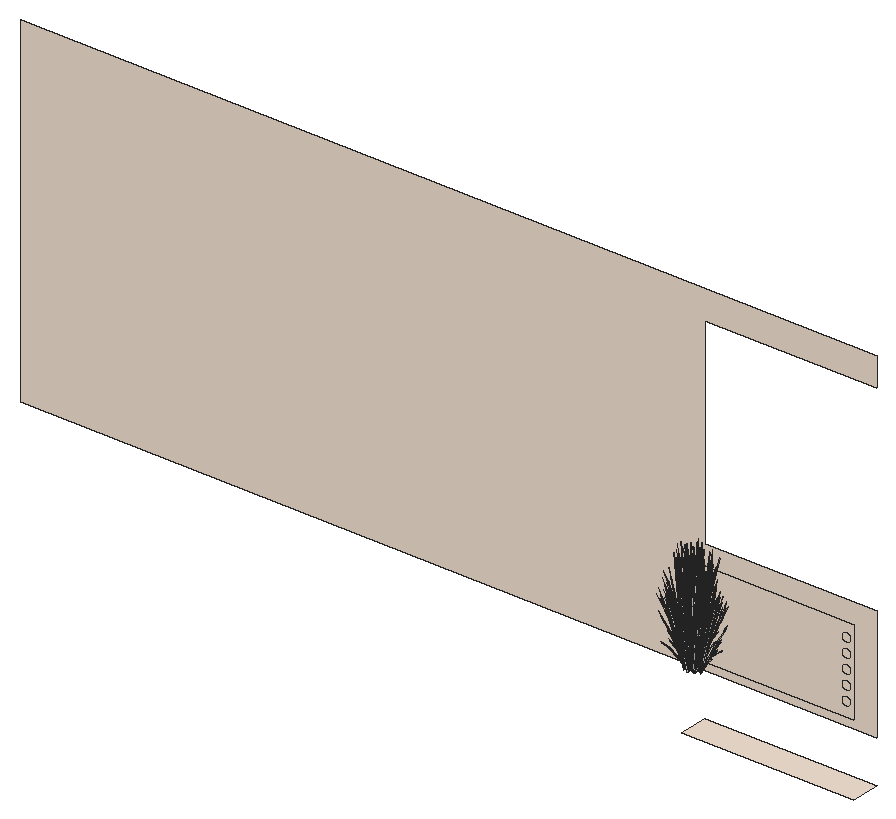
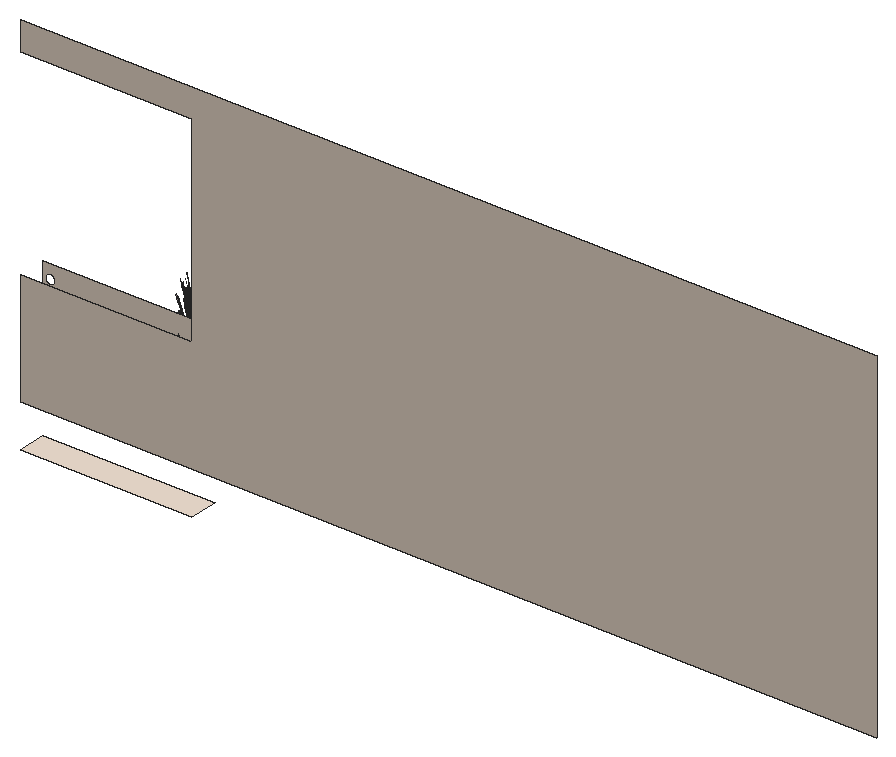
# SketchUp Ruby script. Lengths in inches.
U = 1.inch
M = Sketchup.active_model
def pt(a) = Geom::Point3d.new(a.map { |v| v * U })
def face(e, loops, mat)
  f = e.add_face(loops[0].map { |a| pt(a) })
  loops[1..].each { |l| e.add_face(l.map { |a| pt(a) }).erase! }
  f.material = f.back_material = mat if mat
  f
end
# faces: each face lists its corners as indices into pts; further lists are holes
def faces(e, pts, list, mat = nil) = list.each { |f| face(e, (f[0].is_a?(Array) ? f : [f]).map { |l| l.map { |i| pts[i] } }, mat) }
# xy, xz, yz: faces in a plane at the given z, y or x. An outline is a flat list of corners, or four numbers for a rectangle; further outlines are holes
def ring(l) = l.size == 4 ? [[l[0], l[1]], [l[2], l[1]], [l[2], l[3]], [l[0], l[3]]] : l.each_slice(2).to_a
def flat(e, list, mat, &to3) = list.each { |f| face(e, (f[0].is_a?(Array) ? f : [f]).map { |l| ring(l).map { |u, v| to3.(u, v) } }, mat) }
def xy(e, z, list, mat = nil) = flat(e, list, mat) { |x, y| [x, y, z] }
def xz(e, y, list, mat = nil) = flat(e, list, mat) { |x, z| [x, y, z] }
def yz(e, x, list, mat = nil) = flat(e, list, mat) { |y, z| [x, y, z] }
def lines(e, pts, list) = list.each { |a, b| e.add_line(pt(pts[a]), pt(pts[b])) }
# prism: a flat outline (further loops are holes) pulled along v
def prism(e, loops, v, mat = nil)
  f = face(e, loops, mat); d = Geom::Vector3d.new(v.map { |x| x * U })
  f.pushpull(f.normal.samedirection?(d) ? d.length : -d.length)
end
def box(e, o, s, mat = nil) = prism(e, [[o, [o[0] + s[0], o[1], o[2]], [o[0] + s[0], o[1] + s[1], o[2]], [o[0], o[1] + s[1], o[2]]]], [0, 0, s[2]], mat)
def at(x, y, z, deg = 0) = Geom::Transformation.translation(pt([x, y, z])) * Geom::Transformation.rotation(ORIGIN, Z_AXIS, deg.degrees)
def axes(o, x, y, z) = Geom::Transformation.new([*x, 0, *y, 0, *z, 0, *pt(o).to_a, 1])
def part(name) = M.definitions.add(name)
# library, detail: a bought-in or finely detailed component or shape, given as its bounding box
def library(name, o, s) = part(name).tap { |d| box(d.entities, o, s) }
def detail(e, o, s) = box(e.add_group.entities, o, s)
def put(e, d, t, mat = nil) = e.add_instance(d, t).tap { |i| i.material = mat if mat }
def group(e, t, mat = nil) = e.add_group.tap { |g| g.transformation = t; g.material = mat if mat }.entities
root = M.entities
M.materials.add("C01_Vanilla_Cream").color = [244, 228, 212]
M.materials.add("LightPink_Translucent").color = [144, 107, 117]
M.materials["LightPink_Translucent"].alpha = 0.75
c1 = part("blade")
p = [[2.15,0.21,22],[0,0.17,0],[0.09,0.45,0],[2.18,0.31,22],[2.29,0.31,22],[0.38,0.45,0],
  [2.48,0.24,33],[2.49,0.24,33],[2.48,0.22,33]]
faces(c1.entities,p,[[0,1,2,3],[4,5,2,3],[6,3,4,7],[8,0,3,6]])
c2 = part("seeds")
p = [[0.3,-0.1,1.38],[-0.01,-0.03,1.59],[-0.01,-0.03,0.03],[0.14,-0.07,-0.07],[0.29,-0.03,3],[0.15,0.01,3.11]]
faces(c2.entities,p,[[0,1,2,3],[1,0,4,5]],"LightPink_Translucent")
c3 = part("blade with seeds")
put(c3.entities,c1,at(0,0,0))
put(c3.entities,c2,axes([2.4,0.25,30.99],[1.5799,-0.05474,1.17369],[-0.12525,1.92788,0.29478],[-0.07173,-0.02425,1.56792]))
xy(root,282,[[288,468,360,480]],"C01_Vanilla_Cream")
xz(root,468,[[[288,312,360,348],[357,340,356.48,340.07,356,340.27,355.59,340.59,355.27,341,355.07,341.48,355,342,355.07,342.52,355.27,343,355.59,343.41,356,343.73,356.48,343.93,357,344,357.52,343.93,358,343.73,358.41,343.41,358.73,343,358.93,342.52,359,342,358.93,341.48,358.73,341,358.41,340.59,358,340.27,357.52,340.07],[357,334,356.48,334.07,356,334.27,355.59,334.59,355.27,335,355.07,335.48,355,336,355.07,336.52,355.27,337,355.59,337.41,356,337.73,356.48,337.93,357,338,357.52,337.93,358,337.73,358.41,337.41,358.73,337,358.93,336.52,359,336,358.93,335.48,358.73,335,358.41,334.59,358,334.27,357.52,334.07],[357,328,356.48,328.07,356,328.27,355.59,328.59,355.27,329,355.07,329.48,355,330,355.07,330.52,355.27,331,355.59,331.41,356,331.73,356.48,331.93,357,332,357.52,331.93,358,331.73,358.41,331.41,358.73,331,358.93,330.52,359,330,358.93,329.48,358.73,329,358.41,328.59,358,328.27,357.52,328.07],[357,322,356.48,322.07,356,322.27,355.59,322.59,355.27,323,355.07,323.48,355,324,355.07,324.52,355.27,325,355.59,325.41,356,325.73,356.48,325.93,357,326,357.52,325.93,358,325.73,358.41,325.41,358.73,325,358.93,324.52,359,324,358.93,323.48,358.73,323,358.41,322.59,358,322.27,357.52,322.07],[357,316,356.48,316.07,356,316.27,355.59,316.59,355.27,317,355.07,317.48,355,318,355.07,318.52,355.27,319,355.59,319.41,356,319.73,356.48,319.93,357,320,357.52,319.93,358,319.73,358.41,319.41,358.73,319,358.93,318.52,359,318,358.93,317.48,358.73,317,358.41,316.59,358,316.27,357.52,316.07]]],"C01_Vanilla_Cream")
xz(root,480,[[0,300,0,444,360,444,360,432,288,432,288,348,360,348,360,300]],"C01_Vanilla_Cream")
put(root,c3,axes([301.5625,458.53,315.51],[-0.14302,-0.44985,-0.38324],[0.54163,-0.07869,-0.29685],[0.15522,-0.12083,0.7333]))
put(root,c3,axes([299.2,456.98,313.6],[-0.38473,0.28263,-0.02919],[-0.35252,-0.30954,-0.13237],[-0.02482,-0.08771,0.43661]))
put(root,c3,axes([297.29,457.12,315.54],[-0.11979,-0.00348,1.31208],[-0.38137,0.34775,-0.2075],[-0.20349,-0.07106,0.10523]))
put(root,c3,axes([301.82,458.85,315.78],[-0.515,-0.27165,-0.0912],[0.2967,-0.3934,-0.50621],[0.1455,-0.13675,0.76918]))
put(root,c3,axes([299.69,460.33,314.49],[0.48111,0.19866,1.13446],[-0.47133,0.42798,0.44862],[-0.21112,-0.25366,0.95105]))
put(root,c3,axes([298.68,457.65,315.79],[0.08599,0.39682,0.2656],[-0.49155,0.10478,-0.3429],[-0.13203,-0.11372,0.65611]))
put(root,c3,axes([297.17,458.96,313.51],[0,-0.49266,-0.37238],[0.62289,0,0],[0,-0.11221,1.18128]))
put(root,c3,axes([298.91,457.5,313.51],[0.52105,-0.24633,-0.37238],[0.31144,0.44171,0],[0.11867,-0.0561,1.18128]))
put(root,c3,axes([302,458.35,313.94],[-0.19889,-0.01459,1.07251],[-0.20376,-0.39145,-0.23066],[0.24434,-0.11074,0.45856]))
put(root,c3,axes([297.2,457.91,315.82],[0.45978,-0.36358,0.40322],[0.39653,0.38611,0.33247],[-0.21571,-0.06707,0.83437]))
put(root,c3,axes([303.09,458.73,315.53],[-0.07272,-0.00374,1.33037],[-0.30197,-0.40092,-0.12571],[0.12127,-0.13182,0.23543]))
put(root,c3,axes([299.52,458.51,313.54],[0.375,-0.3703,-0.46765],[0.46584,0.33578,-0.12274],[0.15027,-0.09237,1.03225]))
put(root,c3,axes([302.23,457.63,314.07],[-0.18544,0.25079,0.86145],[-0.15939,-0.33694,0.63294],[0.15316,-0.08443,0.18974]))
put(root,c3,axes([301.96,458.57,315.39],[0.48462,-0.07041,-0.2656],[0.12797,0.4025,0.3429],[0.13888,-0.10811,0.65611]))
put(root,c3,axes([297.41,457.9,315.55],[0.02803,-0.37463,0.04823],[0.42332,0.01027,0.37966],[-0.16216,-0.0392,0.57892]))
put(root,c3,axes([298.87,459.16,313.66],[0.27012,-0.44393,-0.33554],[0.56127,0.21365,0.16149],[0,-0.10233,1.07733]))
put(root,c3,axes([297.25,458.02,315.39],[-0.31678,-0.30846,-0.2656],[0.36171,-0.29199,0.3429],[-0.18378,-0.04443,0.65611]))
put(root,c3,axes([299.12,458.94,314],[-0.06488,-0.56215,-0.21822],[0.6757,-0.03399,-0.37502],[0.11898,-0.07488,1.19781]))
put(root,c3,axes([297.44,458.97,313.52],[0.38863,-0.30738,-0.23233],[0.38863,0.30738,0.23233],[0,-0.09901,1.0423]))
put(root,c3,axes([297.28,457.5,313.6],[-0.1606,0.40228,-0.02919],[-0.4943,-0.12375,-0.13237],[-0.07505,-0.0658,0.43661]))
put(root,c3,axes([301.57,458.8125,315.79],[-0.48462,0.07041,0.2656],[-0.12797,-0.4025,-0.3429],[0.13888,-0.10811,0.65611]))
put(root,c3,axes([298.8,459.53,314],[-0.62699,-0.23507,-0.21822],[0.3019,-0.49615,-0.37502],[-0.0197,-0.12182,1.19781]))
put(root,c3,axes([297.02,459.33,313.78],[-0.69617,0,0],[0,-0.55062,-0.38706],[0,-0.12541,1.22783]))
put(root,c3,axes([297.14,458.35,313.94],[0.1087,0.13716,1.07251],[-0.25048,0.37284,-0.23066],[-0.25719,-0.08912,0.45856]))
put(root,c3,axes([299.03,457.7,313.52],[0.51941,0.1219,-0.23233],[-0.13078,0.42928,0.23233],[0.10471,-0.0495,1.0423]))
put(root,c3,axes([297.59,458.23,315.74],[-0.55654,-0.01186,-0.53284],[0.03738,-0.49951,0.0643],[-0.23578,-0.05271,0.75375]))
put(root,c3,axes([302.01,458.75,315.55],[0.3822,0.20719,0.04823],[-0.22252,0.29505,0.37966],[0.12254,-0.09539,0.57892]))
put(root,c3,axes([301.9,458.66,315.55],[0.13808,0.45342,0.36002],[-0.54163,0.07869,0.29685],[0.15963,-0.10664,0.74497]))
put(root,c3,axes([303.36,459.21,315.54],[0.07726,-0.07504,1.31208],[-0.09888,-0.46032,-0.2075],[0.19384,-0.08728,0.10523]))
put(root,c3,axes([297.56,459.1875,313.75],[-0.51786,0.4142,0.23067],[-0.51817,-0.40984,-0.27369],[-0.01808,-0.11762,1.23664]))
put(root,c3,axes([296.83,457.41,315.53],[0.04127,0.04917,1.33037],[-0.19898,0.44196,-0.12571],[-0.20151,0.0032,0.23543]))
put(root,c3,axes([299.21,459.38,313.82],[0.6273,0.23878,0.18048],[-0.3019,0.49615,0.37502],[0,-0.11437,1.20407]))
put(root,c3,axes([298.96,460.05,313.83],[0.14756,-0.58378,-0.17572],[0.69966,0.10176,0.38453],[-0.12225,-0.08062,1.1733]))
put(root,c3,axes([297.4,458.33,315.51],[-0.40426,0.32635,-0.38324],[-0.35404,-0.34474,-0.29685],[-0.2054,-0.04965,0.7333]))
put(root,c3,axes([297.7,458.18,315.79],[0.31678,0.30846,0.2656],[-0.36171,0.29199,-0.3429],[-0.18378,-0.04443,0.65611]))
put(root,c3,axes([296.49,458.76,314.07],[0.35544,-0.03525,0.86145],[-0.22547,0.31061,0.63294],[-0.17565,-0.04659,0.18974]))
put(root,c3,axes([299,459.05,314.04],[-0.60457,0.03041,0.33554],[-0.05467,-0.50484,-0.16149],[0.10823,-0.05117,1.07733]))
put(root,c3,axes([297.61,457.99,315.78],[-0.02981,0.50103,-0.0912],[-0.56442,-0.01369,-0.50621],[-0.21738,-0.0348,0.76918]))
put(root,c3,axes([297.44,459.42,313.86],[0,0.49266,0.37238],[-0.62289,0,0],[0,-0.11221,1.18128]))
put(root,c3,axes([301.84,459.91,315.78],[-0.28012,-0.44611,-0.0912],[0.49717,-0.21923,-0.50621],[0.20951,-0.05886,0.76918]))
put(root,c3,axes([301.8125,459.53,315.51],[0.15083,-0.44814,-0.38324],[0.51712,0.15361,-0.29685],[0.2082,-0.04109,0.7333]))
put(root,c3,axes([301,457.7,313.78],[0.34808,-0.49367,0],[0.58235,0.27531,-0.38706],[0.13264,0.0627,1.22783]))
put(root,c3,axes([296.9,458.68,314.91],[0.23093,-0.01116,1.28532],[-0.15319,0.4836,0.10393],[-0.32909,-0.02991,0.54946]))
put(root,c3,axes([298.91,459.8125,313.66],[-0.33445,-0.41351,-0.33554],[0.50659,-0.29119,0.16149],[-0.10823,-0.05117,1.07733]))
put(root,c3,axes([298.98,459.23,313.77],[0.24206,0.5509,0.34316],[-0.69162,0.19157,0.13466],[0.00845,-0.10123,1.19142]))
put(root,c3,axes([302.37,459.65,313.49],[-0.35858,0.05912,1.06187],[-0.05708,-0.47061,0.06078],[0.25115,-0.07123,0.60425]))
put(root,c3,axes([303.02,459.24,313.7],[-0.34516,-0.31503,-0.04866],[0.37803,-0.28865,-0.22062],[0.10711,-0.02032,0.72768]))
put(root,c3,axes([298.86,459.66,314.04],[-0.27012,0.44393,0.33554],[-0.56127,-0.21365,-0.16149],[0,-0.10233,1.07733]))
put(root,c3,axes([299.85,459.28,313.65],[0,-0.57005,0],[0.69617,0,0],[0,0,1.34592]))
put(root,c3,axes([300.7,457.96,313.86],[-0.52105,-0.24633,0.37238],[0.31144,-0.44171,0],[0.11867,0.0561,1.18128]))
put(root,c3,axes([301.72,459.6875,315.74],[0.48922,-0.21758,-0.53284],[0.27264,0.44789,0.0643],[0.23638,-0.05088,0.75375]))
put(root,c3,axes([298.61,459.97,313.54],[-0.57914,-0.08077,-0.46765],[0.12221,-0.49823,-0.12274],[-0.17283,-0.06037,1.03225]))
put(root,c3,axes([299.52,458.92,313.77],[-0.46162,0.4471,0.34316],[-0.54842,-0.39467,0.13466],[0.11129,-0.04462,1.19142]))
put(root,c3,axes([300.03,459.72,313.72],[-0.51786,-0.42404,-0.04598],[0.51817,-0.4243,0],[-0.01808,-0.01481,1.31678]))
put(root,c3,axes([298.72,458.18,313.86],[-0.16083,0.48962,0.13232],[-0.58854,-0.13856,0.26315],[0.10167,-0.00238,1.20305]))
put(root,c3,axes([301.64,459.77,315.79],[-0.46269,-0.13744,0.2656],[0.13495,-0.40096,-0.3429],[0.18628,-0.03677,0.65611]))
put(root,c3,axes([296.8,459.04,315.55],[0.15729,-0.44921,0.36002],[0.51712,0.15361,0.29685],[-0.20336,0.027,0.74497]))
put(root,c3,axes([298.48,458.58,313.2],[-0.548,0.19724,0.96696],[-0.17442,-0.56594,0.37572],[0.3365,0.00941,1.09981]))
put(root,c3,axes([299.95,458.73,313.96],[0.1074,-0.43968,0.1086],[0.52474,0.07632,-0.3101],[0.0955,0.04515,0.95058]))
put(root,c3,axes([296.76,458.92,315.55],[-0.20448,-0.33592,0.04823],[0.37288,-0.16442,0.37966],[-0.16437,0.03244,0.57892]))
put(root,c3,axes([299.04,459.77,313.77],[0.70367,0.1038,0.34316],[-0.1432,0.58624,0.13466],[-0.10283,-0.05661,1.19142]))
put(root,c3,axes([302.76,459.34,313.12],[-0.0291,-0.0748,1.32257],[0.20181,-0.43752,-0.20205],[0.20357,-0.00629,0.22528]))
put(root,c3,axes([296.75,459.27,313.12],[0.01412,0.07764,1.32257],[-0.28464,0.40547,-0.20205],[-0.20218,-0.02044,0.22528]))
put(root,c3,axes([299.73,458.84,314.04],[-0.33445,-0.41351,0.33554],[0.50659,-0.29119,-0.16149],[0.10823,0.05117,1.07733]))
put(root,c3,axes([298,460.73,313.52],[-0.13078,-0.42928,-0.23233],[0.51941,-0.1219,0.23233],[-0.10471,-0.0495,1.0423]))
put(root,c3,axes([298.66,460.71,313.86],[0.59825,-0.13076,0.13232],[0.14773,0.48663,0.26315],[-0.05336,-0.0709,1.20305]))
put(root,c3,axes([299.9,458.87,314],[0.56211,-0.32708,-0.21822],[0.3738,0.46216,-0.37502],[0.13869,0.04694,1.19781]))
put(root,c3,axes([302.13,459.73,315.39],[0.46269,0.13744,-0.2656],[-0.13495,0.40096,0.3429],[0.18628,-0.03677,0.65611]))
put(root,c3,axes([297.85,460.92,313.51],[-0.52105,-0.24633,-0.37238],[0.31144,-0.44171,0],[-0.11867,-0.0561,1.18128]))
put(root,c3,axes([301.3125,458,313.51],[0.52105,0.24633,-0.37238],[-0.31144,0.44171,0],[0.11867,0.0561,1.18128]))
put(root,c3,axes([296.69,459.09,315.39],[-0.46269,-0.13744,-0.2656],[0.13495,-0.40096,0.3429],[-0.18628,0.03677,0.65611]))
put(root,c3,axes([300.32,459.4,313.65],[0.62289,0,0],[0,0.51004,0],[0,0,1.33805]))
put(root,c3,axes([299.27,460.05,314],[-0.56211,0.32708,-0.21822],[-0.3738,-0.46216,-0.37502],[-0.13869,-0.04694,1.19781]))
put(root,c3,axes([300.5,458.21,313.86],[-0.59825,0.13076,0.13232],[-0.14773,-0.48663,0.26315],[0.05336,0.0709,1.20305]))
put(root,c3,axes([300.87,459.23,314.91],[-0.23093,0.01116,1.28532],[0.15319,-0.4836,0.10393],[0.32909,0.02991,0.54946]))
put(root,c3,axes([301.17,458.18,313.52],[0.13078,0.42928,-0.23233],[-0.51941,0.1219,0.23233],[0.10471,0.0495,1.0423]))
put(root,c3,axes([302.0625,459.9,315.55],[0.20448,0.33592,0.04823],[-0.37288,0.16442,0.37966],[0.16437,-0.03244,0.57892]))
put(root,c3,axes([300.125,459.14,313.79],[-0.70367,-0.1038,0.36899],[0.1432,-0.58624,0.1448],[0.10283,0.05661,1.2811]))
put(root,c3,axes([302.02,459.78,315.55],[-0.15729,0.44921,0.36002],[-0.51712,-0.15361,0.29685],[0.20336,-0.027,0.74497]))
put(root,c3,axes([299.5625,460.59,313.65],[-0.18165,-0.42474,0],[0.51872,-0.14874,0],[0,0,1.15778]))
put(root,c3,axes([299.22,460.1875,313.96],[-0.1074,0.43968,0.1086],[-0.52474,-0.07632,-0.3101],[-0.0955,-0.04515,0.95058]))
put(root,c3,axes([297.18,459.05,315.79],[0.46269,0.13744,0.2656],[-0.13495,0.40096,-0.3429],[-0.18628,0.03677,0.65611]))
put(root,c3,axes([300.24,460.53,313.64],[0.5845,-0.16716,-0.14398],[0.20539,0.48152,0.00006],[0.06452,-0.01848,1.30423]))
put(root,c3,axes([300.44,460.73,313.86],[0.16083,-0.48962,0.13232],[0.58854,0.13856,0.26315],[-0.10167,0.00238,1.20305]))
put(root,c3,axes([300.3125,459.62,313.66],[0.38863,0.31822,0],[-0.38863,0.31822,0],[0,0,1.2695]))
put(root,c3,axes([298.1,459.02,314.51],[0.15825,-0.07127,1.32798],[0.05457,0.4976,0.10393],[-0.34278,0.06603,0.47463]))
put(root,c3,axes([301.36,459.48,313.86],[-0.43742,-0.35886,0.13232],[0.44081,-0.34807,0.26315],[-0.04831,0.07329,1.20305]))
put(root,c3,axes([300.55,458.94,313.54],[0.57914,0.08077,-0.46765],[-0.12221,0.49823,-0.12274],[0.17283,0.06037,1.03225]))
put(root,c3,axes([303.11,459.8125,314.07],[-0.34399,0.08133,0.86145],[0.16192,-0.33614,0.63294],[0.18249,0.023,0.18974]))
put(root,c3,axes([299.43,460.78,313.65],[-0.56127,-0.22118,0],[0.27012,-0.45959,0],[0,0,1.2203]))
put(root,c3,axes([299.9,460.19,313.85],[-0.54364,-0.39653,-0.18894],[0.45745,-0.44527,0.41347],[-0.14639,0.04639,1.26162]))
put(root,c3,axes([298.47,460.95,313.86],[0.52105,0.24633,0.37238],[-0.31144,0.44171,0],[-0.11867,-0.0561,1.18128]))
put(root,c3,axes([300.31,459.25,314.04],[0.27012,-0.44393,0.33554],[0.56127,0.21365,-0.16149],[0,0.10233,1.07733]))
put(root,c3,axes([302.95,461.23,315.53],[-0.05034,-0.04313,1.33037],[0.11012,-0.46232,-0.12571],[0.1983,-0.02954,0.23543]))
put(root,c3,axes([296.4,459.36,315.54],[-0.09091,0.06396,1.31208],[0.00773,0.46734,-0.2075],[-0.20839,0.06078,0.10523]))
put(root,c3,axes([300.2,459.5,313.72],[0,0.56976,-0.04228],[-0.69617,0,0],[0,0.01791,1.34526]))
put(root,c3,axes([297.01,459.3,315.51],[-0.15083,0.44814,-0.38324],[-0.51712,-0.15361,-0.29685],[-0.2082,0.04109,0.7333]))
put(root,c3,axes([296.99,458.91,315.78],[0.28012,0.44611,-0.0912],[-0.49717,0.21923,-0.50621],[-0.20951,0.05886,0.76918]))
put(root,c3,axes([300.25,459.1,313.66],[0.33445,0.41351,-0.33554],[-0.50659,0.29119,0.16149],[0.10823,0.05117,1.07733]))
put(root,c3,axes([302.51,460.85,314.95],[-0.10656,-0.41414,-0.02619],[0.50364,-0.09521,-0.11874],[0.10517,0.02626,0.39164]))
put(root,c3,axes([298.17,461.21,313.78],[-0.34808,0.49367,0],[-0.58235,-0.27531,-0.38706],[-0.13264,-0.0627,1.22783]))
put(root,c3,axes([301.21,460.84,315.78],[0.02981,-0.50103,-0.0912],[0.56442,0.01369,-0.50621],[0.21738,0.0348,0.76918]))
put(root,c3,axes([301.72,459.5,313.86],[0,-0.49266,0.37238],[0.62289,0,0],[0,0.11221,1.18128]))
put(root,c3,axes([300.16,459.87,314.04],[0.60457,-0.03041,0.33554],[0.05467,0.50484,-0.16149],[-0.10823,0.05117,1.07733]))
put(root,c3,axes([300.54,459.35,313.96],[0.51872,-0.14368,0.1086],[0.18165,0.41027,-0.3101],[0,0.09029,0.95058]))
put(root,c3,axes([301.12,460.64,315.79],[-0.31678,-0.30846,0.2656],[0.36171,-0.29199,-0.3429],[0.18378,0.04443,0.65611]))
put(root,c3,axes([299.625,460.11,313.66],[-0.60457,0.03041,-0.33554],[-0.05467,-0.50484,0.16149],[-0.10823,0.05117,1.07733]))
put(root,c3,axes([302.47,460.35,313.94],[-0.13408,-0.12117,1.07251],[0.17446,-0.40083,-0.23066],[0.27128,0.0543,0.45856]))
put(root,c3,axes([300.07,460.79,313.65],[0.56127,0.22118,0],[-0.27012,0.45959,0],[0,0,1.31215]))
put(root,c3,axes([301.7,460.54,315.54],[0.11943,-0.00833,1.31208],[0.32759,-0.38275,-0.2075],[0.21244,0.05052,0.10523]))
put(root,c3,axes([300.29,461.28,313.64],[-0.34375,-0.4954,-0.03857],[0.58235,-0.27531,0.38706],[-0.1435,0.04717,1.22723]))
put(root,c3,axes([300.17,460.08,313.96],[0.41131,0.296,0.1086],[-0.34309,0.33395,-0.3101],[-0.0955,0.04515,0.95058]))
put(root,c3,axes([296.92,460.16,315.55],[-0.13808,-0.45342,0.36002],[0.54163,-0.07869,0.29685],[-0.15963,0.10664,0.74497]))
put(root,c3,axes([296.82,460.07,315.55],[-0.3822,-0.20719,0.04823],[0.22252,-0.29505,0.37966],[-0.12254,0.09539,0.57892]))
put(root,c3,axes([296.99,459.53,314.91],[0.19317,-0.10421,1.28532],[0.16263,0.48153,0.10393],[-0.30326,0.10883,0.54946]))
put(root,c3,axes([301.24,460.6,315.74],[0.55654,0.01186,-0.53284],[-0.03738,0.49951,0.0643],[0.23578,0.05271,0.75375]))
put(root,c3,axes([300.61,461,313.86],[0.52105,-0.24633,0.37238],[0.31144,0.44171,0],[-0.11867,0.0561,1.18128]))
put(root,c3,axes([299.87,460.61,313.72],[0.24206,0.56598,-0.04509],[-0.69162,0.19832,0],[0.00845,0.01976,1.2913]))
put(root,c3,axes([300.14,461.22,313.52],[-0.51941,-0.1219,-0.23233],[0.13078,-0.42928,0.23233],[-0.10471,0.0495,1.0423]))
put(root,c3,axes([296.39,460.35,313.94],[0.19348,0.04044,1.07251],[0.1247,0.41309,-0.23066],[-0.26282,0.07733,0.45856]))
put(root,c3,axes([297.26,460.01,315.79],[0.48462,-0.07041,0.2656],[0.12797,0.4025,-0.3429],[-0.13888,0.10811,0.65611]))
put(root,c3,axes([302.15,459.58,313.78],[0.69617,0,0],[0,0.55062,-0.38706],[0,0.12541,1.22783]))
put(root,c3,axes([295.39,459.83,315.53],[0.07105,0.01321,1.33037],[0.2198,0.43529,-0.12571],[-0.14545,0.11425,0.23543]))
put(root,c3,axes([301.87,459.86,313.65],[-0.69582,-0.00394,-0.03732],[0,-0.55062,0.37457],[-0.02187,0.12535,1.18764]))
put(root,c3,axes([300.36,459.38,314],[0.62699,0.23507,-0.21822],[-0.3019,0.49615,-0.37502],[0.0197,0.12182,1.19781]))
put(root,c3,axes([295.99,461.21,314.07],[0.23202,-0.22328,0.86145],[0.09155,0.35348,0.63294],[-0.16768,0.06329,0.18974]))
put(root,c3,axes([301.57,460.8,315.39],[0.31678,0.30846,-0.2656],[-0.36171,0.29199,0.3429],[0.18378,0.04443,0.65611]))
put(root,c3,axes([301.72,459.94,313.52],[-0.38863,0.30738,-0.23233],[-0.38863,-0.30738,0.23233],[0,0.09901,1.0423]))
put(root,c3,axes([300.05,459.97,314],[0.06488,0.56215,-0.21822],[-0.6757,0.03399,-0.37502],[-0.11898,0.07488,1.19781]))
put(root,c3,axes([301.41,460.92,315.55],[-0.02803,0.37463,0.04823],[-0.42332,-0.01027,0.37966],[0.16216,0.0392,0.57892]))
put(root,c3,axes([300.3,459.75,313.66],[-0.27012,0.44393,-0.33554],[-0.56127,-0.21365,0.16149],[0,0.10233,1.07733]))
put(root,c3,axes([296.86,460.25,315.39],[-0.48462,0.07041,-0.2656],[-0.12797,-0.4025,0.3429],[-0.13888,0.10811,0.65611]))
put(root,c3,axes([301.45,460.8,315.55],[-0.41051,0.32462,0.36002],[-0.35404,-0.34474,0.29685],[0.1926,0.05988,0.74497]))
put(root,c3,axes([296.16,461.15,316.23],[0.49129,0.13151,-0.04866],[-0.15113,0.40475,-0.22062],[-0.08035,0.06145,0.72768]))
put(root,c3,axes([299.64,460.4,313.54],[-0.375,0.3703,-0.46765],[-0.46584,-0.33578,-0.12274],[-0.15027,0.09237,1.03225]))
put(root,c3,axes([300.14,461.18,315.79],[-0.08599,-0.39682,0.2656],[0.49155,-0.10478,-0.3429],[0.13203,0.11372,0.65611]))
put(root,c3,axes([300.31,461.03,313.75],[0.697,0.16013,0.23067],[-0.17437,0.57237,-0.27369],[-0.11536,0.07164,1.23664]))
put(root,c3,axes([300.26,461.41,313.51],[-0.52105,0.24633,-0.37238],[-0.31144,-0.44171,0],[-0.11867,0.0561,1.18128]))
put(root,c3,axes([301.99,459.96,313.51],[0,0.49266,-0.37238],[-0.62289,0,0],[0,0.11221,1.18128]))
put(root,c3,axes([300.43,460.01,314.91],[-0.2068,-0.08488,1.28532],[0.42797,-0.35609,0.10393],[0.26673,0.16064,0.54946]))
put(root,c3,axes([300.47,458.89,315.36],[-0.48108,-0.25598,1.03712],[0.50798,-0.39855,0.44749],[0.15521,0.24018,1.00248]))
put(root,c3,axes([297.01,459.97,315.78],[0.515,0.27165,-0.0912],[-0.2967,0.3934,-0.50621],[-0.1455,0.13675,0.76918]))
put(root,c3,axes([301.2,460.98,314.07],[-0.31347,-0.14166,0.86145],[0.40476,-0.14393,0.63294],[0.10917,0.12192,0.18974]))
put(root,c3,axes([300.1,461.38,315.78],[0.33176,-0.4217,-0.0912],[0.48044,0.24295,-0.50621],[0.16701,0.11914,0.76918]))
put(root,c3,axes([297.7,459.85,314.91],[0.13906,-0.15138,1.28532],[0.35111,0.40859,0.10393],[-0.24082,0.18608,0.54946]))
put(root,c3,axes([297.26,460.3,315.51],[0.14302,0.44985,-0.38324],[-0.54163,0.07869,-0.29685],[-0.15522,0.12083,0.7333]))
put(root,c3,axes([297.91,460.8125,315.79],[0.3767,-0.25939,0.2656],[0.3566,0.29618,-0.3429],[-0.05426,0.15048,0.65611]))
put(root,c3,axes([300.73,461.34,313.78],[0.34808,0.49367,0],[-0.58235,0.27531,-0.38706],[-0.13264,0.0627,1.22783]))
put(root,c3,axes([299.66,461.73,315.53],[0.00165,-0.05965,1.33037],[0.47711,-0.26315,-0.12571],[0.16572,0.09393,0.23543]))
put(root,c3,axes([301.29,461.5,313.12],[0.04056,-0.07113,1.32257],[0.51066,-0.20948,-0.20205],[0.15482,0.10842,0.22528]))
put(root,c3,axes([300.4375,459.38,314.13],[-0.01521,-0.46386,1.05954],[0.68831,0.12024,0.44862],[-0.1628,0.25382,1.00012]))
put(root,c3,axes([300.61,459.89,313.57],[0.20414,0.45107,-0.51909],[-0.58805,0.16245,-0.13624],[0.02256,0.15274,1.1458]))
put(root,c3,axes([297.57,461.05,315.55],[-0.45752,-0.02296,0.04823],[0.01254,-0.34663,0.37966],[-0.04787,0.13278,0.57892]))
put(root,c3,axes([296.6,461.44,313.12],[0.07468,0.04922,1.32257],[0.12663,0.45605,-0.20205],[-0.16551,0.09725,0.22528]))
put(root,c3,axes([297.72,461.08,315.55],[-0.39645,-0.33614,0.36002],[0.42102,-0.2899,0.29685],[-0.07313,0.15771,0.74497]))
put(root,c3,axes([300.49,461.17,315.51],[0.54938,-0.11711,-0.38324],[0.0961,0.44351,-0.29685],[0.14756,0.1271,0.7333]))
put(root,c3,axes([298.97,461.24,315.79],[0.16784,-0.37886,0.2656],[0.48968,0.1105,-0.3429],[0.0449,0.15254,0.65611]))
put(root,c3,axes([301.25,461.62,314],[-0.35702,-0.01545,0.78795],[0.23577,-0.32816,0.43504],[0.14104,0.11659,0.61808]))
put(root,c3,axes([300.22,461.54,315.55],[-0.25304,0.31296,0.04823],[-0.36033,-0.18221,0.37966],[0.11649,0.10034,0.57892]))
put(root,c3,axes([299.625,462.59,316.23],[0.38473,-0.28263,-0.04866],[0.35252,0.30954,-0.22062],[0.02482,0.08771,0.72768]))
put(root,c3,axes([300.33,461.45,315.55],[-0.55374,0.11306,0.36002],[-0.0961,-0.44351,0.29685],[0.13023,0.13071,0.74497]))
put(root,c3,axes([297.59,460.23,314.91],[0.10366,-0.16934,1.28532],[0.43488,0.35044,0.10393],[-0.19618,0.21841,0.54946]))
put(root,c3,axes([300.08,460.83,313.94],[0.00982,-0.16331,1.07251],[0.4695,-0.18242,-0.23066],[0.14493,0.19547,0.45856]))
put(root,c3,axes([298.82,461.58,315.55],[-0.41024,0.16744,0.04823],[-0.2008,-0.30532,0.37966],[0.03962,0.13459,0.57892]))
put(root,c3,axes([297.71,461.18,315.39],[-0.3767,0.25939,-0.2656],[-0.3566,-0.29618,0.3429],[-0.05426,0.15048,0.65611]))
put(root,c3,axes([296.42,461.1,315.54],[-0.01384,0.09749,1.31208],[0.39274,0.33916,-0.2075],[-0.10282,0.16039,0.10523]))
put(root,c3,axes([297.67,460.88,316.05],[0.61188,0.02441,-0.10123],[-0.01672,0.46217,-0.56189],[-0.0425,0.178,0.85379]))
put(root,c3,axes([298.8,461.4,315.78],[0.54481,-0.22937,-0.0912],[0.26773,0.4071,-0.50621],[0.07188,0.17155,0.76918]))
put(root,c3,axes([298.96,461.55,315.8],[-0.54859,-0.1288,0.39962],[0.18759,-0.42344,0.32951],[0.03297,0.16652,0.82692]))
put(root,c3,axes([297.95,462.1875,314.07],[-0.01441,-0.29294,0.86145],[0.36003,0.20894,0.63294],[-0.07081,0.13963,0.18974]))
put(root,c3,axes([298.9,461.49,313.12],[0.0901,-0.02681,1.32257],[0.54199,0.14755,-0.20205],[0.01585,0.1663,0.22528]))
put(root,c3,axes([298.09,461.06,315.75],[0.39855,0.33102,-0.4254],[-0.42102,0.2899,-0.32951],[-0.06064,0.16819,0.81396]))
put(root,c3,axes([297.66,461.55,314.12],[0.50577,-0.08724,0.04881],[0.11627,0.35148,-0.64728],[-0.03206,0.17792,0.5802]))
put(root,c3,axes([299.27,461.38,315.51],[0.54728,0.1235,-0.38324],[-0.18759,0.42344,-0.29685],[0.05018,0.17048,0.7333]))
put(root,c3,axes([299.58,460.5,314.91],[-0.12726,-0.15818,1.28532],[0.58807,-0.13317,0.10393],[0.13291,0.24832,0.54946]))
put(root,c3,axes([299.02,461.64,315.39],[-0.16784,0.37886,-0.2656],[-0.48968,-0.1105,0.3429],[0.0449,0.15254,0.65611]))
put(root,c3,axes([297.97,460.91,316],[-0.01449,0.45571,-0.59145],[-0.61002,-0.03061,0.07138],[-0.06438,0.19306,0.83667]))
put(root,c3,axes([296.37,462.1,315.53],[0.06316,-0.02974,1.33037],[0.52204,0.19785,-0.12571],[-0.01227,0.16473,0.23543]))
put(root,c3,axes([298.54,460.58,314.91],[-0.01363,-0.18909,1.28532],[0.5906,0.12544,0.10393],[-0.03653,0.26947,0.54946]))
put(root,c3,axes([299.07,461.3,315.74],[0.26572,0.40059,-0.53284],[-0.54698,0.22325,0.0643],[0.06214,0.19355,0.75375]))
put(root,c3,axes([297.53,461.93,313.94],[0.17569,-0.07772,1.07251],[0.43377,0.23434,-0.23066],[-0.12911,0.20277,0.45856]))
put(root,c3,axes([298.68,462.31,315.54],[0.07057,0.07933,1.31208],[0.56952,0.03117,-0.2075],[0.05727,0.17496,0.10523]))
put(root,c3,axes([297.76,461.55,314.52],[0.01223,-0.25433,1.15759],[0.55017,0.13434,0.15997],[-0.04767,0.27105,0.54661]))
